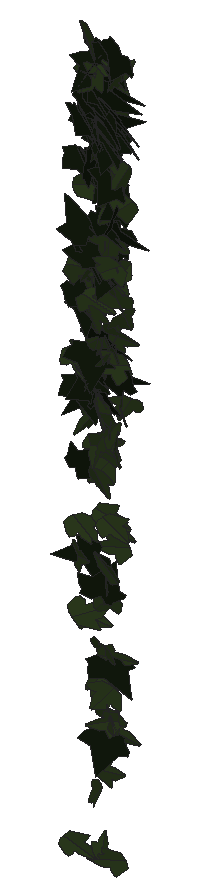
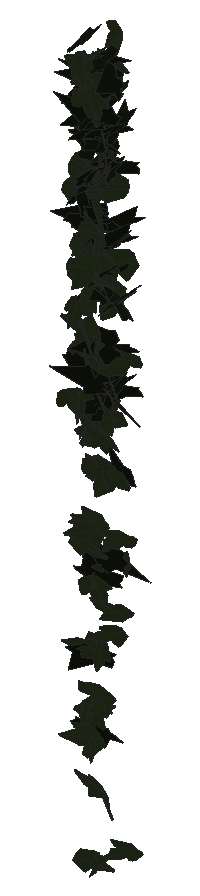
# SketchUp Ruby script. Lengths in inches.
U = 1.inch
M = Sketchup.active_model
def pt(a) = Geom::Point3d.new(a.map { |v| v * U })
def face(e, loops, mat)
  f = e.add_face(loops[0].map { |a| pt(a) })
  loops[1..].each { |l| e.add_face(l.map { |a| pt(a) }).erase! }
  f.material = f.back_material = mat if mat
  f
end
# faces: each face lists its corners as indices into pts; further lists are holes
def faces(e, pts, list, mat = nil) = list.each { |f| face(e, (f[0].is_a?(Array) ? f : [f]).map { |l| l.map { |i| pts[i] } }, mat) }
# xy, xz, yz: faces in a plane at the given z, y or x. An outline is a flat list of corners, or four numbers for a rectangle; further outlines are holes
def ring(l) = l.size == 4 ? [[l[0], l[1]], [l[2], l[1]], [l[2], l[3]], [l[0], l[3]]] : l.each_slice(2).to_a
def flat(e, list, mat, &to3) = list.each { |f| face(e, (f[0].is_a?(Array) ? f : [f]).map { |l| ring(l).map { |u, v| to3.(u, v) } }, mat) }
def xy(e, z, list, mat = nil) = flat(e, list, mat) { |x, y| [x, y, z] }
def xz(e, y, list, mat = nil) = flat(e, list, mat) { |x, z| [x, y, z] }
def yz(e, x, list, mat = nil) = flat(e, list, mat) { |y, z| [x, y, z] }
def lines(e, pts, list) = list.each { |a, b| e.add_line(pt(pts[a]), pt(pts[b])) }
# prism: a flat outline (further loops are holes) pulled along v
def prism(e, loops, v, mat = nil)
  f = face(e, loops, mat); d = Geom::Vector3d.new(v.map { |x| x * U })
  f.pushpull(f.normal.samedirection?(d) ? d.length : -d.length)
end
def box(e, o, s, mat = nil) = prism(e, [[o, [o[0] + s[0], o[1], o[2]], [o[0] + s[0], o[1] + s[1], o[2]], [o[0], o[1] + s[1], o[2]]]], [0, 0, s[2]], mat)
def at(x, y, z, deg = 0) = Geom::Transformation.translation(pt([x, y, z])) * Geom::Transformation.rotation(ORIGIN, Z_AXIS, deg.degrees)
def axes(o, x, y, z) = Geom::Transformation.new([*x, 0, *y, 0, *z, 0, *pt(o).to_a, 1])
def part(name) = M.definitions.add(name)
# library, detail: a bought-in or finely detailed component or shape, given as its bounding box
def library(name, o, s) = part(name).tap { |d| box(d.entities, o, s) }
def detail(e, o, s) = box(e.add_group.entities, o, s)
def put(e, d, t, mat = nil) = e.add_instance(d, t).tap { |i| i.material = mat if mat }
def group(e, t, mat = nil) = e.add_group.tap { |g| g.transformation = t; g.material = mat if mat }.entities
root = M.entities
M.materials.add("1026 AP 7946 SUNNY SIDE UP").color = [254, 231, 186]
M.materials.add("efeu1").color = [18, 25, 13]
M.materials.add("efeu2").color = [43, 57, 29]
c1 = part("ivyleaf_9")
p = [[1.54,2.16,1.25],[1.36,2.04,1.19],[-0.21,0.99,0.68],[-0.71,1.11,0.82],[-0.85,0.86,0.67],[-0.8,0.17,0.21],
  [-0.9,-0.01,0.1],[-0.67,-0.16,-0.02],[-0.08,-0.08,-0.05],[-0.03,-0.6,-0.4],[0.65,-0.88,-0.66],[0.83,-0.6,-0.49],
  [1.29,-0.42,-0.43],[1.8125,-0.07,-0.26],[1.21,0.44,0.15]]
faces(c1.entities,p,[[0,1,2,3,4,5,6,7,8,9,10,11,12,13,14]],"efeu1")
c2 = part("ivyleaf_10")
p = [[0,0.5,-0.03],[-0.0625,2.02,-0.43],[-0.19,2.01,-0.46],[-0.54,1.05,-0.29],[-0.52,0.625,-0.18],[-0.83,0.76,-0.28],
  [-1.16,0.64,-0.33],[-1.15,0.33,-0.24],[-0.77,-0.39,0.02],[-0.3,-0.51,0.16],[0.04,-0.48,0.23],[-0.02,2.01,-0.4375],
  [-0.06,2.01,-0.43],[0.04,-0.49,0.23],[0.67,-0.49,0.14],[1.38,0.36,-0.2],[1.375,0.51,-0.24],[0.81,0.65,-0.19],
  [0.62,0.59,-0.15],[0.6,1.09,-0.28],[0.5,1.23,-0.31]]
faces(c2.entities,p,[[0,1,2,3,4,5,6,7,8,9,10],[11,12,0,13,14,15,16,17,18,19,20]],"efeu2")
put(root,c1,axes([107.89,212.19,258.05],[-0.1131,0.12619,0.20317],[0.13242,-0.17776,0.14832],[0.3425,0.1104,0.00974]),"1026 AP 7946 SUNNY SIDE UP")
put(root,c1,axes([107.87,212.19,262.09],[0.14668,-0.2192,-0.11431],[-0.02754,0.11113,-0.24342],[0.38444,0.0916,0.02617]),"1026 AP 7946 SUNNY SIDE UP")
put(root,c1,axes([108.1875,212.31,259.85],[-0.35882,0.09717,-0.08066],[0.09934,-0.05208,-0.2548],[-0.16985,-0.23575,0.02137]),"1026 AP 7946 SUNNY SIDE UP")
put(root,c2,axes([107.86,212.28,256.76],[0.21857,0.14499,0.1332],[0.1682,0.07438,-0.20528],[-0.25395,0.17405,-0.02132]),"1026 AP 7946 SUNNY SIDE UP")
put(root,c1,axes([108.01,212.18,261.87],[-0.16357,0.2364,-0.02471],[-0.00388,0.02657,0.26609],[0.37383,0.10371,-0.00805]),"1026 AP 7946 SUNNY SIDE UP")
put(root,c1,axes([107.97,212.3,265.83],[-0.09065,-0.12473,0.2281],[0.01465,-0.22862,-0.1311],[0.4003,-0.01988,0.05645]),"1026 AP 7946 SUNNY SIDE UP")
put(root,c1,axes([108.35,212.26,256.22],[-0.04038,-0.04395,-0.26022],[-0.32726,-0.14424,0.04686],[-0.23476,0.20864,-0.02056]),"1026 AP 7946 SUNNY SIDE UP")
put(root,c2,axes([108.02,212.52,258.2],[-0.31745,-0.11707,-0.08209],[0.1241,0.02082,-0.23938],[0.18419,-0.2158,0.01979]),"1026 AP 7946 SUNNY SIDE UP")
put(root,c1,axes([108.08,212.24,266.88],[0.06448,0.13704,0.25006],[0.11989,0.22965,-0.14597],[-0.42047,0.0865,-0.00327]),"1026 AP 7946 SUNNY SIDE UP")
put(root,c2,axes([107.97,212.34,267.9],[-0.22142,0.18839,-0.13883],[0.10984,-0.11714,-0.24266],[-0.34828,-0.15671,0.01173]),"1026 AP 7946 SUNNY SIDE UP")
put(root,c1,axes([108.25,212.05,263.48],[-0.29313,-0.16169,0.07746],[0.06948,0.06486,0.25384],[-0.27227,0.19063,-0.01862]),"1026 AP 7946 SUNNY SIDE UP")
put(root,c1,axes([107.92,212.39,262.75],[0.13145,-0.17101,-0.15681],[-0.011,0.15907,-0.18834],[0.3588,0.06753,0.05168]),"1026 AP 7946 SUNNY SIDE UP")
put(root,c2,axes([108.03,212.48,260.54],[-0.34452,-0.10245,0.07616],[0.09069,0.05186,0.24849],[-0.17736,0.22554,-0.02088]),"1026 AP 7946 SUNNY SIDE UP")
put(root,c2,axes([107.89,212.18,256.05],[-0.10926,0.06123,0.21458],[0.29664,-0.09048,0.09186],[0.16789,0.19971,-0.02266]),"1026 AP 7946 SUNNY SIDE UP")
put(root,c1,axes([107.95,212.39,265.06],[-0.10009,-0.20008,-0.15994],[0.11041,0.13865,-0.2145],[0.38146,-0.09263,0.02012]),"1026 AP 7946 SUNNY SIDE UP")
put(root,c1,axes([107.91,212.49,264.96],[0.22311,-0.20117,-0.01239],[-0.02166,0.0036,-0.25341],[0.31605,0.14226,-0.00862]),"1026 AP 7946 SUNNY SIDE UP")
put(root,c2,axes([107.89,212,249.7],[0.14991,0.0996,0.17576],[0.20888,0.10705,-0.14069],[-0.22888,0.16293,-0.01328]),"1026 AP 7946 SUNNY SIDE UP")
put(root,c2,axes([108.0625,212.55,264.86],[-0.09056,0.2331,-0.05774],[0.01395,-0.05689,-0.24764],[-0.3772,-0.05806,0.0047]),"1026 AP 7946 SUNNY SIDE UP")
put(root,c1,axes([108.05,212.6,265.85],[-0.1366,-0.24231,-0.03133],[0.02138,0.02597,-0.26501],[0.38315,-0.08784,0.00362]),"1026 AP 7946 SUNNY SIDE UP")
put(root,c2,axes([107.98,212.13,260.67],[0.34476,0.12277,0.07169],[0.10633,0.01999,-0.2583],[-0.19416,0.22896,-0.01415]),"1026 AP 7946 SUNNY SIDE UP")
put(root,c2,axes([108,212.24,264.42],[-0.0112,-0.01219,0.27456],[0.11735,0.25595,0.01561],[-0.40287,0.07489,-0.00309]),"1026 AP 7946 SUNNY SIDE UP")
put(root,c2,axes([107.95,212.38,254.67],[-0.09595,-0.09308,-0.19049],[0.28394,0.06928,-0.09719],[0.15764,-0.18144,0.05911]),"1026 AP 7946 SUNNY SIDE UP")
put(root,c1,axes([108.18,212.32,259.93],[-0.11485,-0.12578,0.2216],[-0.15409,-0.19241,-0.15081],[0.3613,-0.12204,0.00612]),"1026 AP 7946 SUNNY SIDE UP")
put(root,c2,axes([108.12,212.55,253.12],[0.12136,0.18706,-0.0657],[-0.03381,-0.06126,-0.2088],[-0.30946,0.08005,-0.00295]),"1026 AP 7946 SUNNY SIDE UP")
put(root,c1,axes([107.96,212.19,260.28],[0.31645,-0.16224,-0.02175],[-0.04444,-0.00298,-0.26553],[0.25321,0.20224,-0.01942]),"1026 AP 7946 SUNNY SIDE UP")
put(root,c2,axes([108.32,212.56,258.37],[-0.306,-0.00756,0.11345],[-0.16967,-0.03445,-0.19899],[0.03692,-0.22096,0.02582]),"1026 AP 7946 SUNNY SIDE UP")
put(root,c2,axes([108.1875,212.36,265.11],[0.08627,-0.23921,-0.12527],[0.00394,0.1232,-0.25058],[0.42096,0.04787,0.02802]),"1026 AP 7946 SUNNY SIDE UP")
put(root,c1,axes([108.05,212.21,261.84],[-0.00648,-0.24039,0.05737],[-0.00218,-0.05704,-0.24802],[0.38849,-0.00433,-0.00043]),"1026 AP 7946 SUNNY SIDE UP")
put(root,c1,axes([107.96,212.68,267.47],[0.1159,-0.23198,0.10391],[0.05133,-0.09684,-0.25131],[0.39526,0.0806,0.00217]),"1026 AP 7946 SUNNY SIDE UP")
put(root,c2,axes([108.1875,212.61,262.66],[0.04839,-0.18951,0.14116],[0.02179,-0.13757,-0.19847],[0.36807,0.03306,-0.00681]),"1026 AP 7946 SUNNY SIDE UP")
put(root,c1,axes([108.05,212.23,259.98],[-0.13402,-0.20826,-0.12819],[0.11678,0.10185,-0.22962],[0.36216,-0.10991,0.0266]),"1026 AP 7946 SUNNY SIDE UP")
put(root,c1,axes([108.01,212.24,263.23],[0.15091,-0.2303,-0.02944],[-0.01512,0.02554,-0.25688],[0.36435,0.09645,0.00153]),"1026 AP 7946 SUNNY SIDE UP")
put(root,c2,axes([107.99,212.01,262.73],[-0.07753,-0.08231,-0.27506],[0.31659,0.17683,-0.09359],[0.30358,-0.20543,0.02736]),"1026 AP 7946 SUNNY SIDE UP")
put(root,c2,axes([108.07,212.61,259.74],[0.24088,-0.0937,0.13444],[0.15725,-0.08644,-0.18463],[0.19857,0.18211,-0.01687]),"1026 AP 7946 SUNNY SIDE UP")
put(root,c1,axes([108.03,212.19,266.49],[0.25663,-0.17731,-0.08265],[-0.05405,0.07547,-0.24654],[0.30055,0.16498,0.02624]),"1026 AP 7946 SUNNY SIDE UP")
put(root,c1,axes([108.03,212.53,265.56],[0.03755,-0.14353,0.21306],[0.05667,-0.20448,-0.15109],[0.39283,0.04322,0.00143]),"1026 AP 7946 SUNNY SIDE UP")
put(root,c2,axes([108.23,212.3125,259.32],[0.01207,-0.14329,0.23339],[0.03207,-0.22649,-0.14908],[0.42136,0.02134,0.00466]),"1026 AP 7946 SUNNY SIDE UP")
put(root,c2,axes([108.26,212.23,260.31],[0.14218,-0.24099,-0.02418],[-0.01658,0.01965,-0.26503],[0.38016,0.09099,-0.00251]),"1026 AP 7946 SUNNY SIDE UP")
put(root,c2,axes([108.22,212.37,265.18],[0.01496,-0.213,-0.17789],[0.06553,0.17069,-0.21506],[0.42493,-0.01883,0.03943]),"1026 AP 7946 SUNNY SIDE UP")
put(root,c1,axes([108.07,212.38,263.14],[0.06047,-0.27182,0.04492],[0.00504,-0.04514,-0.28306],[0.43324,0.03847,-0.00298]),"1026 AP 7946 SUNNY SIDE UP")
put(root,c2,axes([108.05,212.61,265.71],[0.04639,-0.07287,0.25563],[0.27583,-0.17843,-0.07638],[0.29964,0.17553,0.03074]),"1026 AP 7946 SUNNY SIDE UP")
put(root,c2,axes([108.3,212.56,262.87],[-0.35551,-0.06715,0.02147],[-0.02145,-0.02825,-0.24197],[0.10863,-0.22532,0.02249]),"1026 AP 7946 SUNNY SIDE UP")
put(root,c2,axes([108.26,212.47,260.83],[0.02627,-0.18125,0.14256],[0.01612,-0.13905,-0.18832],[0.35919,0.01949,-0.00197]),"1026 AP 7946 SUNNY SIDE UP")
put(root,c1,axes([108.33,212,265.16],[0.06396,0.00864,-0.29355],[-0.31687,0.20453,-0.02205],[0.31717,0.2026,0.03717]),"1026 AP 7946 SUNNY SIDE UP")
put(root,c1,axes([108.4375,212.11,263.03],[-0.31953,-0.1784,0.07986],[0.07667,0.06332,0.27853],[-0.29675,0.20845,-0.01403]),"1026 AP 7946 SUNNY SIDE UP")
put(root,c2,axes([108.29,212.18,262.76],[0.04469,-0.25122,-0.0865],[0.02223,0.08434,-0.25895],[0.4152,0.02252,0.02318]),"1026 AP 7946 SUNNY SIDE UP")
put(root,c1,axes([108.14,212.58,264.98],[0.07767,-0.22872,-0.07861],[-0.02406,0.07343,-0.24062],[0.37772,0.05171,0.00084]),"1026 AP 7946 SUNNY SIDE UP")
put(root,c1,axes([108.4,212.37,267.21],[-0.32274,-0.14386,0.04992],[-0.04723,-0.04278,-0.25784],[0.23439,-0.20671,0.01677]),"1026 AP 7946 SUNNY SIDE UP")
put(root,c2,axes([108.375,212.25,250.9],[0.15014,-0.18526,-0.09467],[-0.08203,0.07517,-0.21397],[0.31389,0.10826,-0.01064]),"1026 AP 7946 SUNNY SIDE UP")
put(root,c1,axes([108.02,212.46,261.02],[0.3333,-0.0435,0.10995],[0.15223,-0.05496,-0.22097],[0.09899,0.23098,-0.03039]),"1026 AP 7946 SUNNY SIDE UP")
put(root,c2,axes([108.36,212.12,267.13],[0.34851,-0.11727,-0.05625],[-0.08565,0.01218,-0.25783],[0.184,0.22779,-0.01348]),"1026 AP 7946 SUNNY SIDE UP")
put(root,c2,axes([108.44,212.4,263.96],[0.16241,-0.18112,-0.19952],[-0.12663,0.17545,-0.21339],[0.39602,0.13038,0.01359]),"1026 AP 7946 SUNNY SIDE UP")
put(root,c2,axes([108.05,212.34,262.5],[-0.011,0.03469,0.27069],[0.38004,-0.10655,0.02051],[0.17026,0.24007,-0.0283]),"1026 AP 7946 SUNNY SIDE UP")
put(root,c2,axes([108.34,212.4,249.39],[0.04505,0.16917,-0.13211],[0.02846,0.12795,0.17749],[0.33349,-0.03377,0.0027]),"1026 AP 7946 SUNNY SIDE UP")
put(root,c2,axes([108.32,212.08,261.78],[-0.35256,0.04155,-0.03728],[0.05115,-0.02377,-0.23439],[-0.07022,-0.22591,0.01643]),"1026 AP 7946 SUNNY SIDE UP")
put(root,c1,axes([108.28,212.2,260.77],[-0.19536,-0.22329,-0.05799],[0.0632,0.04049,-0.26255],[0.35604,-0.12971,0.01479]),"1026 AP 7946 SUNNY SIDE UP")
put(root,c2,axes([108.1,212.04,254.87],[0.23553,-0.0163,-0.20375],[0.3027,0.07165,0.14461],[0.07517,-0.23745,0.0561]),"1026 AP 7946 SUNNY SIDE UP")
put(root,c1,axes([108.15,212.55,259.58],[0.08549,-0.13753,0.20481],[0.08792,-0.19191,-0.15305],[0.37084,0.07721,-0.01093]),"1026 AP 7946 SUNNY SIDE UP")
put(root,c1,axes([108.17,212.41,262.27],[0.33779,-0.11203,0.01676],[0.00828,-0.02632,-0.24883],[0.17796,0.21388,-0.02023]),"1026 AP 7946 SUNNY SIDE UP")
put(root,c2,axes([108.41,212.57,264.85],[0.30014,-0.14783,-0.04901],[-0.05075,0.0346,-0.2484],[0.23844,0.19345,0.00881]),"1026 AP 7946 SUNNY SIDE UP")
put(root,c2,axes([108.33,212.36,260.69],[-0.14904,0.18915,-0.09598],[0.05205,-0.08873,-0.21826],[-0.32819,-0.09997,0.00897]),"1026 AP 7946 SUNNY SIDE UP")
put(root,c2,axes([108.44,212.17,260.89],[0.15097,-0.22056,-0.05437],[-0.02753,0.04857,-0.24751],[0.35508,0.09754,0.00393]),"1026 AP 7946 SUNNY SIDE UP")
put(root,c2,axes([108.5625,212.49,266.38],[-0.38493,0.04337,0.10706],[-0.16936,-0.01964,-0.25366],[-0.05042,-0.26512,0.0347]),"1026 AP 7946 SUNNY SIDE UP")
put(root,c2,axes([108.46,212.26,254.14],[-0.32792,0.1282,0.0292],[-0.05495,-0.00432,-0.25121],[-0.19875,-0.21032,0.02127]),"1026 AP 7946 SUNNY SIDE UP")
put(root,c2,axes([108.34,212.52,263.12],[-0.20087,0.16569,0.16378],[0.18353,-0.10858,0.21383],[0.30975,0.17178,-0.02048]),"1026 AP 7946 SUNNY SIDE UP")
put(root,c2,axes([108.49,212.3,258.23],[0.3209,-0.06662,-0.07178],[-0.11221,0.00396,-0.2204],[0.10127,0.21549,-0.01676]),"1026 AP 7946 SUNNY SIDE UP")
put(root,c2,axes([108.49,212.5,266.81],[0.34902,0.07908,-0.10517],[-0.14441,-0.0473,-0.24268],[-0.14353,0.23989,-0.01157]),"1026 AP 7946 SUNNY SIDE UP")
put(root,c1,axes([108.49,212.67,264.51],[-0.23601,-0.16334,0.10514],[-0.01323,-0.12478,-0.21725],[0.30334,-0.13253,0.07233]),"1026 AP 7946 SUNNY SIDE UP")
put(root,c2,axes([108.3,212.07,262.08],[-0.16534,-0.12446,-0.18066],[0.27343,0.06437,-0.15473],[0.19737,-0.19344,0.06302]),"1026 AP 7946 SUNNY SIDE UP")
put(root,c1,axes([108.3,212.59,267.42],[0.11454,-0.24325,-0.03863],[0.00617,0.03882,-0.26092],[0.38663,0.07145,0.01561]),"1026 AP 7946 SUNNY SIDE UP")
put(root,c1,axes([108.33,212.45,259.6],[0.33388,-0.11911,-0.03994],[0.06941,0.00116,0.24976],[-0.18398,-0.21572,0.02175]),"1026 AP 7946 SUNNY SIDE UP")
put(root,c1,axes([108.26,212.66,265.35],[0.01693,-0.14092,0.22083],[0.1499,-0.19782,-0.13955],[0.37561,0.0853,0.04574]),"1026 AP 7946 SUNNY SIDE UP")
put(root,c1,axes([108.24,212.57,265.58],[0.10899,-0.18914,0.16604],[0.10912,-0.14709,-0.20806],[0.37634,0.09743,0.01224]),"1026 AP 7946 SUNNY SIDE UP")
put(root,c2,axes([108.59,212.16,262.53],[-0.29967,0.10963,0.08138],[-0.12052,0.02347,-0.2257],[-0.17428,-0.20473,0.01615]),"1026 AP 7946 SUNNY SIDE UP")
put(root,c2,axes([108.42,212.58,252.1],[-0.18664,0.14266,-0.1139],[0.0847,-0.09931,-0.19077],[-0.27169,-0.12896,0.01877]),"1026 AP 7946 SUNNY SIDE UP")
put(root,c1,axes([108.48,212.55,265.55],[-0.33022,-0.10227,-0.11814],[0.18496,0.01644,-0.23813],[0.15439,-0.23844,0.0326]),"1026 AP 7946 SUNNY SIDE UP")
put(root,c2,axes([108.4,212.17,258.82],[0.30809,-0.11797,0.10103],[0.11263,-0.07153,-0.2349],[0.21406,0.20742,-0.02181]),"1026 AP 7946 SUNNY SIDE UP")
put(root,c2,axes([108.65,212.36,260.72],[-0.28611,0.1252,-0.11377],[-0.12373,0.08093,0.2271],[0.23236,0.19726,-0.01915]),"1026 AP 7946 SUNNY SIDE UP")
put(root,c2,axes([108.44,212.15,258.1],[-0.30721,0.07864,-0.08178],[0.10356,-0.04923,-0.2163],[-0.14256,-0.20523,0.01911]),"1026 AP 7946 SUNNY SIDE UP")
put(root,c2,axes([108.77,212.05,259.62],[-0.14192,0.02477,0.22112],[-0.33617,0.02231,-0.0952],[-0.04755,-0.23164,0.01309]),"1026 AP 7946 SUNNY SIDE UP")
put(root,c2,axes([108.27,212.56,251.18],[0.0699,-0.05156,-0.21001],[0.28201,-0.09891,0.06557],[-0.17175,-0.18339,0.02221]),"1026 AP 7946 SUNNY SIDE UP")
put(root,c1,axes([108.38,212.53,264.82],[0.07634,-0.22434,-0.10383],[-0.01941,0.09908,-0.23574],[0.38541,0.04943,0.00869]),"1026 AP 7946 SUNNY SIDE UP")
put(root,c2,axes([108.61,212.3,253.17],[0.35388,-0.05556,-0.09518],[-0.14721,0.00385,-0.23812],[0.08321,0.24313,-0.01648]),"1026 AP 7946 SUNNY SIDE UP")
put(root,c1,axes([108.18,212.25,266.78],[0.3193,-0.0239,0.1993],[0.29722,-0.04492,-0.21023],[0.07577,0.27695,-0.01522]),"1026 AP 7946 SUNNY SIDE UP")
put(root,c2,axes([108.53,212.6,262.02],[0.01553,-0.20133,0.13032],[0.05577,-0.12509,-0.20682],[0.37067,0.02726,0.02566]),"1026 AP 7946 SUNNY SIDE UP")
put(root,c1,axes([108.39,212.35,266.65],[0.08856,-0.25682,-0.02079],[-0.01525,0.01704,-0.27069],[0.4046,0.05685,-0.00565]),"1026 AP 7946 SUNNY SIDE UP")
put(root,c2,axes([108.53,212.06,259.68],[-0.13868,0.23603,0.00895],[-0.01739,0.00371,-0.25938],[-0.3709,-0.08843,0.00881]),"1026 AP 7946 SUNNY SIDE UP")
put(root,c2,axes([108.77,212.38,249.39],[0.10524,-0.00228,-0.21265],[-0.32341,-0.01907,-0.0686],[-0.02742,0.21615,-0.00702]),"1026 AP 7946 SUNNY SIDE UP")
put(root,c2,axes([108.28,212.59,263.5],[0.19597,-0.01436,0.23672],[0.34766,-0.06572,-0.12811],[0.1014,0.25309,-0.01825]),"1026 AP 7946 SUNNY SIDE UP")
put(root,c2,axes([108.74,212.15,255.39],[-0.29575,-0.00642,0.12835],[-0.19139,-0.04024,-0.19162],[0.04325,-0.22201,0.02968]),"1026 AP 7946 SUNNY SIDE UP")
put(root,c1,axes([108.77,212.39,263.64],[-0.00386,-0.0339,-0.26135],[-0.16817,-0.23015,0.03142],[-0.3653,0.10631,-0.0117]),"1026 AP 7946 SUNNY SIDE UP")
put(root,c2,axes([108.59,212.37,260.7],[-0.01085,-0.22697,0.01757],[0.00372,-0.01842,-0.23402],[0.35804,-0.00668,0.00296]),"1026 AP 7946 SUNNY SIDE UP")
put(root,c2,axes([108.6,212.55,267.13],[-0.13746,-0.24992,-0.02163],[0.02551,0.01505,-0.27247],[0.39336,-0.08831,0.01011]),"1026 AP 7946 SUNNY SIDE UP")
put(root,c2,axes([108.4375,212.34,258.83],[-0.26595,0.01269,-0.13554],[0.19311,-0.0642,-0.16932],[-0.07714,-0.20448,0.04343]),"1026 AP 7946 SUNNY SIDE UP")
put(root,c1,axes([108.47,212.57,265.7],[-0.03676,-0.24356,-0.04436],[-0.00472,0.04214,-0.25172],[0.38851,-0.02253,-0.00726]),"1026 AP 7946 SUNNY SIDE UP")
put(root,c2,axes([108.32,212.47,257.04],[0.11914,0.06429,0.20809],[0.2893,0.08581,-0.09891],[-0.16442,0.19756,-0.02326]),"1026 AP 7946 SUNNY SIDE UP")
put(root,c2,axes([108.8,212.48,256.42],[0.13847,-0.04093,-0.20493],[-0.31437,0.0192,-0.09525],[0.05406,0.21648,-0.02898]),"1026 AP 7946 SUNNY SIDE UP")
put(root,c2,axes([108.64,212.56,261.25],[0.13926,-0.20417,-0.05662],[-0.05492,0.04337,-0.22854],[0.32742,0.09411,-0.01425]),"1026 AP 7946 SUNNY SIDE UP")
put(root,c1,axes([108.26,212.45,265.875],[0.0593,-0.02877,0.26952],[0.38983,-0.08534,-0.04695],[0.13971,0.25034,0.01662]),"1026 AP 7946 SUNNY SIDE UP")
put(root,c1,axes([108.38,212.37,266.13],[0.15036,-0.21386,0.09464],[0.04742,-0.08842,-0.24171],[0.36366,0.09995,-0.00761]),"1026 AP 7946 SUNNY SIDE UP")
put(root,c1,axes([108.28,212.4375,260.14],[0.17709,0.00671,0.22609],[0.34345,-0.02807,-0.11478],[0.03449,0.24504,-0.01789]),"1026 AP 7946 SUNNY SIDE UP")
put(root,c2,axes([108.58,212.34,252.66],[-0.33358,0.06556,-0.0541],[0.06541,-0.04306,-0.22717],[-0.11517,-0.21436,0.02767]),"1026 AP 7946 SUNNY SIDE UP")
put(root,c2,axes([108.65,212.64,263.23],[-0.04212,-0.21287,0.11059],[-0.00334,-0.10902,-0.22141],[0.37572,-0.02483,0.01043]),"1026 AP 7946 SUNNY SIDE UP")
put(root,c2,axes([108.87,212.32,260.625],[0.15073,-0.0232,-0.24534],[-0.37507,-0.02765,-0.09635],[-0.02695,0.2551,-0.03123]),"1026 AP 7946 SUNNY SIDE UP")
put(root,c2,axes([108.73,212.42,262.51],[0.17445,0.19674,0.11792],[-0.1139,-0.08889,0.23147],[0.33836,-0.13135,0.01713]),"1026 AP 7946 SUNNY SIDE UP")
put(root,c2,axes([108.56,212.2,258.83],[-0.16955,-0.19832,0.10581],[0.05855,0.09776,0.23276],[-0.3471,0.11337,-0.01242]),"1026 AP 7946 SUNNY SIDE UP")
put(root,c2,axes([108.55,212.45,262.5],[-0.24726,-0.13556,-0.11039],[0.17639,0.0288,-0.20845],[0.20568,-0.18766,0.04606]),"1026 AP 7946 SUNNY SIDE UP")
put(root,c1,axes([108.51,212.63,263.19],[0.02398,-0.21655,0.12878],[0.0016,-0.12642,-0.22427],[0.39413,0.01369,-0.00692]),"1026 AP 7946 SUNNY SIDE UP")
put(root,c2,axes([108.44,212.52,256.81],[-0.18867,-0.02473,-0.19029],[0.29258,-0.00711,-0.12367],[0.01175,-0.22003,0.02408]),"1026 AP 7946 SUNNY SIDE UP")
put(root,c2,axes([108.68,212.27,262.76],[-0.24905,-0.20055,-0.03866],[-0.05478,-0.01877,0.26267],[-0.31577,0.16143,-0.01507]),"1026 AP 7946 SUNNY SIDE UP")
put(root,c1,axes([108.51,212.1,263.98],[0.20166,-0.18456,-0.12668],[-0.08068,0.11226,-0.23002],[0.33832,0.13678,0.02065]),"1026 AP 7946 SUNNY SIDE UP")
put(root,c2,axes([108.86,212.09,255.94],[-0.21532,0.0874,-0.17029],[-0.21775,0.09117,0.16788],[0.19857,0.19475,-0.00055]),"1026 AP 7946 SUNNY SIDE UP")
put(root,c2,axes([108.74,212.07,255.55],[0,-0.04929,-0.21881],[-0.05107,0.20974,-0.04898],[0.33858,0.03164,-0.00739]),"1026 AP 7946 SUNNY SIDE UP")
put(root,c2,axes([108.8,212.21,252.61],[0.0259,0.0079,-0.23289],[-0.23052,-0.1723,-0.01821],[-0.27096,0.14734,-0.00676]),"1026 AP 7946 SUNNY SIDE UP")
put(root,c1,axes([108.64,212.27,262.77],[-0.14539,-0.22461,0.07233],[-0.01821,-0.07237,-0.2501],[0.37019,-0.09177,0.0161]),"1026 AP 7946 SUNNY SIDE UP")
put(root,c1,axes([108.625,212.04,255.49],[-0.29851,0.04502,0.16006],[0.22974,-0.05417,0.2001],[0.10826,0.2391,0.01671]),"1026 AP 7946 SUNNY SIDE UP")
put(root,c2,axes([108.58,212.27,259.14],[-0.22008,0.12484,0.14182],[0.18501,-0.07273,0.19175],[0.22512,0.18182,-0.01894]),"1026 AP 7946 SUNNY SIDE UP")
put(root,c2,axes([108.75,212.18,263.42],[-0.3511,-0.07262,0.02709],[-0.02835,-0.0305,-0.24088],[0.11832,-0.2228,0.02268]),"1026 AP 7946 SUNNY SIDE UP")
put(root,c2,axes([108.53,212.39,256.92],[0.17554,0.12686,0.14476],[0.15747,0.09788,-0.17331],[-0.25162,0.14975,-0.00748]),"1026 AP 7946 SUNNY SIDE UP")
put(root,c2,axes([108.4375,212.51,252.24],[-0.15387,-0.00439,-0.23635],[0.3588,-0.02791,-0.09989],[-0.03769,-0.24783,0.01397]),"1026 AP 7946 SUNNY SIDE UP")
put(root,c2,axes([108.72,212.29,252.47],[-0.16559,0.20114,0.03329],[0.03515,-0.02345,0.23358],[0.31811,0.10729,-0.00848]),"1026 AP 7946 SUNNY SIDE UP")
put(root,c1,axes([108.92,212.34,260.13],[0.05754,-0.03544,0.26418],[-0.23012,0.21104,0.05276],[-0.33614,-0.15055,0.00911]),"1026 AP 7946 SUNNY SIDE UP")
put(root,c1,axes([108.74,212.17,252.24],[-0.35805,-0.10035,-0.1064],[0.16489,0.01535,-0.25485],[0.15426,-0.24933,0.02544]),"1026 AP 7946 SUNNY SIDE UP")
put(root,c1,axes([108.37,212.13,266.69],[0.20282,-0.04417,-0.2434],[0.33937,0.13874,0.09558],[0.16546,-0.23042,0.10232]),"1026 AP 7946 SUNNY SIDE UP")
put(root,c2,axes([108.86,212.42,259.57],[-0.1265,0.12387,0.19061],[-0.19146,0.13934,-0.15041],[-0.29203,-0.14501,0.01604]),"1026 AP 7946 SUNNY SIDE UP")
put(root,c1,axes([108.7,212.28,264.72],[-0.12816,-0.18813,0.16439],[-0.01488,-0.16664,-0.20697],[0.38871,-0.06841,0.04628]),"1026 AP 7946 SUNNY SIDE UP")
put(root,c2,axes([108.6,212.28,266.95],[0.15567,0.12063,-0.26808],[0.23381,0.21466,0.16163],[0.3868,-0.17831,0.01018]),"1026 AP 7946 SUNNY SIDE UP")
put(root,c2,axes([108.92,212.08,262.95],[0.27359,-0.01405,-0.16234],[-0.24585,0.01968,-0.17964],[0.03713,0.23386,0.00675]),"1026 AP 7946 SUNNY SIDE UP")
put(root,c2,axes([108.8,212.45,267.08],[0.0146,-0.26161,-0.07186],[0.02044,0.06866,-0.26884],[0.42464,0.00569,0.01541]),"1026 AP 7946 SUNNY SIDE UP")
put(root,c1,axes([108.57,212.45,265.98],[0.2802,-0.17831,0.00846],[-0.00832,-0.0183,-0.25924],[0.28063,0.1775,-0.01613]),"1026 AP 7946 SUNNY SIDE UP")
put(root,c1,axes([108.48,212.26,263.61],[0.28025,-0.02568,0.1699],[0.24334,-0.0655,-0.18303],[0.09891,0.23393,-0.0311]),"1026 AP 7946 SUNNY SIDE UP")
put(root,c2,axes([108.93,212.2,262.11],[-0.35865,-0.0446,-0.08091],[-0.12628,0.00406,0.2387],[-0.06422,0.24111,-0.01752]),"1026 AP 7946 SUNNY SIDE UP")
put(root,c1,axes([108.74,212.27,263.76],[0.07609,0.15119,0.21484],[-0.11926,-0.19351,0.1622],[0.38593,-0.08961,0.00776]),"1026 AP 7946 SUNNY SIDE UP")
put(root,c2,axes([108.91,212.59,259.6875],[-0.24513,-0.12948,0.07943],[-0.06839,-0.06865,-0.20778],[0.22749,-0.16016,0.02313]),"1026 AP 7946 SUNNY SIDE UP")
put(root,c1,axes([108.74,212.5,267.5],[-0.07887,-0.19483,0.18679],[-0.0132,-0.18437,-0.20631],[0.41946,-0.04243,0.02863]),"1026 AP 7946 SUNNY SIDE UP")
put(root,c2,axes([108.56,212.46,261.125],[-0.10234,-0.0357,0.23624],[0.36465,0.00349,0.06833],[-0.02065,0.23854,0.03578]),"1026 AP 7946 SUNNY SIDE UP")
put(root,c2,axes([108.97,212.36,264.24],[-0.18795,-0.11686,0.23656],[-0.10318,-0.23169,-0.15756],[0.39274,-0.11679,0.07181]),"1026 AP 7946 SUNNY SIDE UP")
put(root,c2,axes([108.8125,212.55,264.85],[-0.04229,-0.15679,0.22112],[0.09196,-0.21481,-0.15473],[0.40887,0.0321,0.05767]),"1026 AP 7946 SUNNY SIDE UP")
put(root,c1,axes([108.79,212.49,264.18],[0.09518,-0.12271,-0.22387],[0.16201,-0.19059,0.13977],[-0.35636,-0.11942,0.00375]),"1026 AP 7946 SUNNY SIDE UP")
put(root,c1,axes([108.68,212.19,253.92],[-0.10934,-0.13707,-0.20096],[0.16452,0.16414,-0.15691],[0.33573,-0.12508,0.01144]),"1026 AP 7946 SUNNY SIDE UP")
put(root,c1,axes([108.62,212.15,266.5],[0.39828,-0.13937,-0.01435],[-0.03599,-0.01444,-0.29692],[0.21716,0.25323,-0.02289]),"1026 AP 7946 SUNNY SIDE UP")
put(root,c2,axes([108.61,212.21,254],[-0.03215,-0.01546,0.23065],[0.28996,0.12713,0.02712],[-0.20137,0.18553,0.00223]),"1026 AP 7946 SUNNY SIDE UP")
put(root,c2,axes([108.85,212.45,261.67],[-0.11205,-0.1906,-0.12424],[0.07122,0.11064,-0.20896],[0.3465,-0.08438,0.00277]),"1026 AP 7946 SUNNY SIDE UP")
put(root,c2,axes([109.01,212.05,258.83],[-0.08575,0.08742,0.25144],[-0.24657,0.18686,-0.10416],[-0.3237,-0.16549,0.01273]),"1026 AP 7946 SUNNY SIDE UP")
